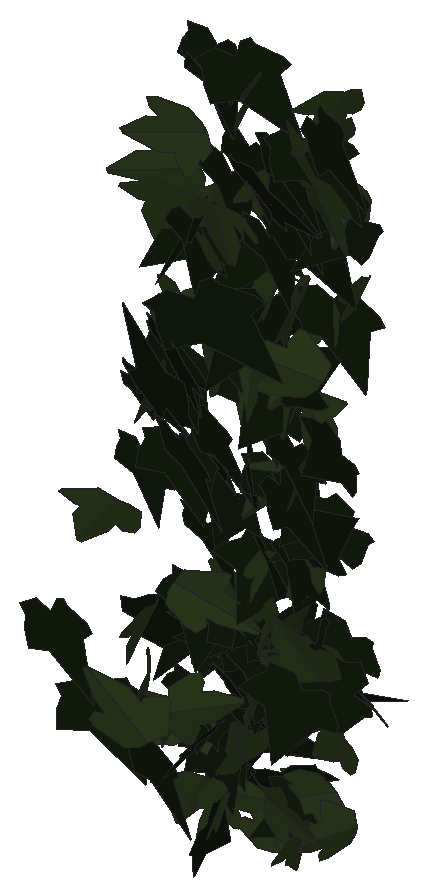
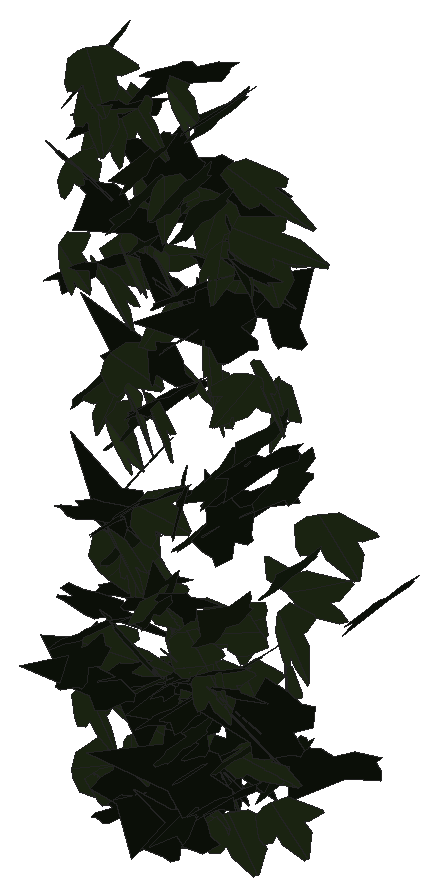
# SketchUp Ruby script. Lengths in inches.
U = 1.inch
M = Sketchup.active_model
def pt(a) = Geom::Point3d.new(a.map { |v| v * U })
def face(e, loops, mat)
  f = e.add_face(loops[0].map { |a| pt(a) })
  loops[1..].each { |l| e.add_face(l.map { |a| pt(a) }).erase! }
  f.material = f.back_material = mat if mat
  f
end
# faces: each face lists its corners as indices into pts; further lists are holes
def faces(e, pts, list, mat = nil) = list.each { |f| face(e, (f[0].is_a?(Array) ? f : [f]).map { |l| l.map { |i| pts[i] } }, mat) }
# xy, xz, yz: faces in a plane at the given z, y or x. An outline is a flat list of corners, or four numbers for a rectangle; further outlines are holes
def ring(l) = l.size == 4 ? [[l[0], l[1]], [l[2], l[1]], [l[2], l[3]], [l[0], l[3]]] : l.each_slice(2).to_a
def flat(e, list, mat, &to3) = list.each { |f| face(e, (f[0].is_a?(Array) ? f : [f]).map { |l| ring(l).map { |u, v| to3.(u, v) } }, mat) }
def xy(e, z, list, mat = nil) = flat(e, list, mat) { |x, y| [x, y, z] }
def xz(e, y, list, mat = nil) = flat(e, list, mat) { |x, z| [x, y, z] }
def yz(e, x, list, mat = nil) = flat(e, list, mat) { |y, z| [x, y, z] }
def lines(e, pts, list) = list.each { |a, b| e.add_line(pt(pts[a]), pt(pts[b])) }
# prism: a flat outline (further loops are holes) pulled along v
def prism(e, loops, v, mat = nil)
  f = face(e, loops, mat); d = Geom::Vector3d.new(v.map { |x| x * U })
  f.pushpull(f.normal.samedirection?(d) ? d.length : -d.length)
end
def box(e, o, s, mat = nil) = prism(e, [[o, [o[0] + s[0], o[1], o[2]], [o[0] + s[0], o[1] + s[1], o[2]], [o[0], o[1] + s[1], o[2]]]], [0, 0, s[2]], mat)
def at(x, y, z, deg = 0) = Geom::Transformation.translation(pt([x, y, z])) * Geom::Transformation.rotation(ORIGIN, Z_AXIS, deg.degrees)
def axes(o, x, y, z) = Geom::Transformation.new([*x, 0, *y, 0, *z, 0, *pt(o).to_a, 1])
def part(name) = M.definitions.add(name)
# library, detail: a bought-in or finely detailed component or shape, given as its bounding box
def library(name, o, s) = part(name).tap { |d| box(d.entities, o, s) }
def detail(e, o, s) = box(e.add_group.entities, o, s)
def put(e, d, t, mat = nil) = e.add_instance(d, t).tap { |i| i.material = mat if mat }
def group(e, t, mat = nil) = e.add_group.tap { |g| g.transformation = t; g.material = mat if mat }.entities
root = M.entities
M.materials.add("1026 AP 7946 SUNNY SIDE UP").color = [254, 231, 186]
M.materials.add("efeu1").color = [18, 25, 13]
M.materials.add("efeu2").color = [43, 57, 29]
c1 = part("ivyleaf_10")
p = [[0,0.5,-0.03],[-0.0625,2.02,-0.43],[-0.19,2.01,-0.46],[-0.54,1.05,-0.29],[-0.52,0.625,-0.18],[-0.83,0.76,-0.28],
  [-1.16,0.64,-0.33],[-1.15,0.33,-0.24],[-0.77,-0.39,0.02],[-0.3,-0.51,0.16],[0.04,-0.48,0.23],[-0.02,2.01,-0.4375],
  [-0.06,2.01,-0.43],[0.04,-0.49,0.23],[0.67,-0.49,0.14],[1.38,0.36,-0.2],[1.375,0.51,-0.24],[0.81,0.65,-0.19],
  [0.62,0.59,-0.15],[0.6,1.09,-0.28],[0.5,1.23,-0.31]]
faces(c1.entities,p,[[0,1,2,3,4,5,6,7,8,9,10],[11,12,0,13,14,15,16,17,18,19,20]],"efeu2")
c2 = part("ivyleaf_9")
p = [[1.54,2.16,1.25],[1.36,2.04,1.19],[-0.21,0.99,0.68],[-0.71,1.11,0.82],[-0.85,0.86,0.67],[-0.8,0.17,0.21],
  [-0.9,-0.01,0.1],[-0.67,-0.16,-0.02],[-0.08,-0.08,-0.05],[-0.03,-0.6,-0.4],[0.65,-0.88,-0.66],[0.83,-0.6,-0.49],
  [1.29,-0.42,-0.43],[1.8125,-0.07,-0.26],[1.21,0.44,0.15]]
faces(c2.entities,p,[[0,1,2,3,4,5,6,7,8,9,10,11,12,13,14]],"efeu1")
put(root,c1,axes([125.9,211.91,280.18],[-0.21426,-0.24961,0.13484],[-0.08049,-0.12264,-0.2934],[0.43686,-0.14502,0.01207]),"1026 AP 7946 SUNNY SIDE UP")
put(root,c2,axes([125.66,211.98,283.87],[0.04707,-0.31543,0.10585],[0.0219,-0.10368,-0.32699],[0.52205,0.03279,0.00417]),"1026 AP 7946 SUNNY SIDE UP")
put(root,c1,axes([126.125,210.66,283.84],[-0.41418,-0.14278,0.1658],[-0.19271,-0.11107,-0.30725],[0.27921,-0.28846,0.03389]),"1026 AP 7946 SUNNY SIDE UP")
put(root,c2,axes([125.74,211.64,285.24],[0.41137,-0.17857,-0.12342],[-0.1051,0.11015,-0.3216],[0.32044,0.26537,0.05296]),"1026 AP 7946 SUNNY SIDE UP")
put(root,c2,axes([125.77,210.97,280.66],[-0.12936,-0.29497,-0.23967],[0.15409,0.2113,-0.31272],[0.56858,-0.12438,0.03022]),"1026 AP 7946 SUNNY SIDE UP")
put(root,c1,axes([126.41,211.85,288.63],[-0.15114,-0.01057,0.36615],[-0.42458,-0.23747,-0.08388],[0.36392,-0.28144,0.0542]),"1026 AP 7946 SUNNY SIDE UP")
put(root,c2,axes([125.875,209.73,282.48],[0.15357,-0.35799,-0.09597],[-0.03239,0.08883,-0.38174],[0.57994,0.09976,0.00409]),"1026 AP 7946 SUNNY SIDE UP")
put(root,c1,axes([126.33,211.76,286.52],[0.1888,-0.21894,-0.27075],[-0.22717,0.21856,-0.25551],[0.48587,0.18726,-0.01426]),"1026 AP 7946 SUNNY SIDE UP")
put(root,c2,axes([126.08,212.02,285.5],[0.04043,-0.33743,-0.16447],[-0.00679,0.15783,-0.34762],[0.58564,0.02512,0.00733]),"1026 AP 7946 SUNNY SIDE UP")
put(root,c1,axes([126.64,211.67,289.35],[0.293,-0.09758,-0.33633],[-0.50379,0.07465,-0.2113],[0.17992,0.36793,-0.04394]),"1026 AP 7946 SUNNY SIDE UP")
put(root,c2,axes([125.82,211.83,281.44],[0.26233,0.01004,0.32465],[0.49231,-0.04681,-0.16952],[0.05774,0.35344,-0.02957]),"1026 AP 7946 SUNNY SIDE UP")
put(root,c1,axes([126.53,211.56,288.33],[-0.53792,-0.12889,0.11284],[-0.1416,-0.07234,-0.37536],[0.22602,-0.35208,0.03339]),"1026 AP 7946 SUNNY SIDE UP")
put(root,c2,axes([126.43,212.14,281.53],[-0.43662,0.03839,-0.16325],[0.22799,-0.08593,-0.2833],[-0.11801,-0.30806,0.05671]),"1026 AP 7946 SUNNY SIDE UP")
put(root,c2,axes([126.15,212.01,285.65],[0.11219,-0.3542,0.13675],[0.0355,-0.1329,-0.37298],[0.59483,0.07474,-0.00354]),"1026 AP 7946 SUNNY SIDE UP")
put(root,c1,axes([126.35,211.99,286.46],[-0.29245,-0.24062,-0.16416],[0.27249,0.05658,-0.29863],[0.3614,-0.23738,0.09232]),"1026 AP 7946 SUNNY SIDE UP")
put(root,c1,axes([126.61,210.85,282.27],[0.08597,-0.37699,0.06829],[0.01345,-0.0679,-0.39283],[0.60231,0.05533,-0.00097]),"1026 AP 7946 SUNNY SIDE UP")
put(root,c1,axes([126.68,210.74,281.45],[0.10564,-0.26469,-0.20128],[-0.03103,0.19428,-0.27916],[0.51497,0.06601,0.02447]),"1026 AP 7946 SUNNY SIDE UP")
put(root,c1,axes([126.67,210.91,285.77],[0.01043,-0.27646,-0.24771],[0.01766,0.23896,-0.28319],[0.57424,-0.00233,0.01321]),"1026 AP 7946 SUNNY SIDE UP")
put(root,c1,axes([126.86,211.43,280.51],[0.30086,0.09889,-0.25801],[-0.33829,-0.12976,-0.22237],[-0.25598,0.28771,-0.00938]),"1026 AP 7946 SUNNY SIDE UP")
put(root,c1,axes([126.8,212.17,282.01],[-0.16875,-0.2955,0.11595],[-0.0092,-0.11874,-0.32279],[0.49807,-0.10231,0.03332]),"1026 AP 7946 SUNNY SIDE UP")
put(root,c2,axes([126.96,211.8,288.01],[-0.52918,-0.07609,0.03235],[-0.03598,-0.04235,-0.35375],[0.12461,-0.33538,0.03523]),"1026 AP 7946 SUNNY SIDE UP")
put(root,c2,axes([126.51,212.28,282.96],[0.09016,-0.29168,0.14703],[0.10212,-0.1334,-0.30499],[0.50146,0.07961,0.03568]),"1026 AP 7946 SUNNY SIDE UP")
put(root,c2,axes([126.65,211.57,284.59],[-0.12958,-0.31232,-0.1472],[0.05934,0.13598,-0.33196],[0.53561,-0.09063,0.00117]),"1026 AP 7946 SUNNY SIDE UP")
put(root,c2,axes([126.66,211.96,282.03],[-0.08444,-0.34733,0.15121],[0.0081,-0.1509,-0.36197],[0.59407,-0.04731,0.02643]),"1026 AP 7946 SUNNY SIDE UP")
put(root,c1,axes([126.96,211.53,279.47],[-0.31475,-0.23428,0.10941],[-0.07714,-0.09903,-0.31694],[0.39793,-0.20451,0.0251]),"1026 AP 7946 SUNNY SIDE UP")
put(root,c1,axes([126.79,211.99,288.28],[-0.10063,-0.3401,-0.03506],[0.15434,0.01297,-0.34313],[0.51449,-0.07041,0.09608]),"1026 AP 7946 SUNNY SIDE UP")
put(root,c1,axes([126.89,212.1,286.9],[0.05887,-0.34036,-0.10486],[0.01883,0.10157,-0.35142],[0.55742,0.03251,0.02295]),"1026 AP 7946 SUNNY SIDE UP")
put(root,c2,axes([126.94,211.55,288.24],[-0.34851,0.15259,-0.2622],[0.29811,-0.17298,-0.27699],[-0.36049,-0.29056,0.02444]),"1026 AP 7946 SUNNY SIDE UP")
put(root,c2,axes([126.56,212.0625,284.15],[0.41505,-0.11879,-0.17574],[0.26803,-0.03222,0.29582],[-0.18555,-0.31226,0.03422]),"1026 AP 7946 SUNNY SIDE UP")
put(root,c2,axes([126.61,210.85,280.17],[0.25311,-0.34619,0.02628],[-0.00276,-0.03109,-0.3932],[0.54605,0.16031,-0.01417]),"1026 AP 7946 SUNNY SIDE UP")
put(root,c2,axes([126.74,211.81,280.67],[-0.05678,-0.28883,0.1652],[0.0277,-0.1644,-0.29888],[0.51998,-0.02278,0.03396]),"1026 AP 7946 SUNNY SIDE UP")
put(root,c1,axes([126.85,211.58,287.78],[-0.41219,0.21266,-0.08037],[0.05824,-0.07932,-0.34608],[-0.35205,-0.26211,0.03684]),"1026 AP 7946 SUNNY SIDE UP")
put(root,c2,axes([126.71,211.98,280.1875],[0.07354,-0.30815,-0.09412],[0.02086,0.09234,-0.31944],[0.50418,0.04112,0.02694]),"1026 AP 7946 SUNNY SIDE UP")
put(root,c2,axes([126.92,212.15,281.8],[-0.36679,-0.21363,-0.04625],[0.10572,-0.00963,-0.32148],[0.32616,-0.23712,0.0522]),"1026 AP 7946 SUNNY SIDE UP")
put(root,c2,axes([126.51,212.05,287.36],[0.42447,-0.00759,0.22204],[0.33911,0.01643,-0.27752],[-0.00681,0.34507,0.02013]),"1026 AP 7946 SUNNY SIDE UP")
put(root,c1,axes([127.18,211.61,285.92],[0.03021,-0.00244,-0.37477],[-0.24899,0.3279,-0.00896],[0.51497,0.15868,0.01766]),"1026 AP 7946 SUNNY SIDE UP")
put(root,c1,axes([127.26,212.04,282.29],[-0.37935,0.0735,0.23987],[-0.37344,0.00281,-0.25487],[-0.08637,-0.33499,0.04843]),"1026 AP 7946 SUNNY SIDE UP")
put(root,c2,axes([126.79,212.12,290.5],[-0.01189,-0.34847,0.07198],[0.00196,-0.07189,-0.35949],[0.55946,-0.00715,0.00279]),"1026 AP 7946 SUNNY SIDE UP")
put(root,c2,axes([126.9,211.66,287.88],[-0.02053,-0.31755,0.21286],[-0.0241,-0.20794,-0.32858],[0.59677,-0.01932,-0.00594]),"1026 AP 7946 SUNNY SIDE UP")
put(root,c2,axes([127.125,212.21,281.9],[-0.31569,-0.24526,0.14014],[-0.07183,-0.13817,-0.32359],[0.43619,-0.20026,0.04814]),"1026 AP 7946 SUNNY SIDE UP")
put(root,c2,axes([126.85,211.99,290.33],[0.07159,-0.33275,0.10543],[0.03972,-0.10169,-0.34641],[0.54684,0.05095,0.01136]),"1026 AP 7946 SUNNY SIDE UP")
put(root,c1,axes([126.9,211.92,281.87],[0.20417,0.23732,0.19125],[0.16186,0.15348,-0.27743],[-0.44387,0.16513,-0.0132]),"1026 AP 7946 SUNNY SIDE UP")
put(root,c2,axes([126.84,211.78,284.9],[0.31395,-0.31377,-0.03146],[-0.03224,0.02103,-0.38297],[0.49439,0.20062,-0.005]),"1026 AP 7946 SUNNY SIDE UP")
put(root,c1,axes([127.24,210.82,281.21],[0.03761,-0.38204,0.05583],[0.00268,-0.05637,-0.39467],[0.60722,0.02391,-0.00171]),"1026 AP 7946 SUNNY SIDE UP")
put(root,c2,axes([127.3125,211.2,280.48],[-0.22647,0.19756,-0.21128],[0.14467,-0.18653,-0.2514],[-0.42509,-0.16873,0.027]),"1026 AP 7946 SUNNY SIDE UP")
put(root,c2,axes([127.59,211.84,281.79],[-0.39332,0.21224,0.11918],[-0.17616,0.04379,-0.33555],[-0.33578,-0.27158,0.03644]),"1026 AP 7946 SUNNY SIDE UP")
put(root,c2,axes([127.23,212.27,287.01],[-0.21043,-0.20198,0.28859],[-0.10601,-0.28058,-0.24226],[0.53408,-0.13528,0.06562]),"1026 AP 7946 SUNNY SIDE UP")
put(root,c1,axes([126.87,211.47,282.4],[0.17157,0.11682,0.33616],[0.43237,0.17793,-0.15963],[-0.33013,0.29375,-0.03437]),"1026 AP 7946 SUNNY SIDE UP")
put(root,c2,axes([127.29,212.24,287.64],[-0.21923,-0.28492,0.14128],[-0.04982,-0.1383,-0.32616],[0.49581,-0.13988,0.0297]),"1026 AP 7946 SUNNY SIDE UP")
put(root,c2,axes([127.15,211.79,280.46],[0.02541,-0.31283,-0.04939],[0.00441,0.04637,-0.32239],[0.4972,0.01558,0.00538]),"1026 AP 7946 SUNNY SIDE UP")
put(root,c2,axes([127.11,212.03,288.7],[0.02188,-0.31138,0.19306],[0.04089,-0.18797,-0.32182],[0.57142,0.02537,0.01564]),"1026 AP 7946 SUNNY SIDE UP")
put(root,c2,axes([127.25,211.9,283.88],[-0.13291,-0.26682,0.21314],[-0.00672,-0.21395,-0.28521],[0.53231,-0.06932,0.04962]),"1026 AP 7946 SUNNY SIDE UP")
put(root,c2,axes([127.58,210.01,286.23],[0.22051,-0.18211,0.37102],[-0.22428,0.33545,0.23326],[-0.59517,-0.19388,0.04956]),"1026 AP 7946 SUNNY SIDE UP")
put(root,c2,axes([127.23,212.11,281.84],[0.00985,-0.31605,-0.07882],[0.00526,0.07479,-0.32519],[0.51064,0.00533,0.00487]),"1026 AP 7946 SUNNY SIDE UP")
put(root,c2,axes([127.24,212.26,280.88],[-0.00424,-0.27285,0.17992],[0.04292,-0.17577,-0.28101],[0.5089,0.01255,0.0252]),"1026 AP 7946 SUNNY SIDE UP")
put(root,c1,axes([127.45,211.34,288.5],[-0.53448,0.08056,-0.02626],[0.02721,-0.03898,-0.35841],[-0.13027,-0.33866,0.03289]),"1026 AP 7946 SUNNY SIDE UP")
put(root,c1,axes([127.76,209.18,281.66],[0.42812,0.09371,0.27639],[-0.42494,-0.02715,0.29273],[0.13561,-0.3809,0.04475]),"1026 AP 7946 SUNNY SIDE UP")
put(root,c2,axes([127.29,212.1875,289.08],[0.08936,-0.32492,0.12848],[0.04398,-0.12357,-0.34048],[0.54652,0.06307,0.00639]),"1026 AP 7946 SUNNY SIDE UP")
put(root,c2,axes([127.32,211.49,280.23],[-0.21941,-0.12673,-0.2633],[0.44049,-0.01094,-0.15247],[0.07917,-0.29036,0.11864]),"1026 AP 7946 SUNNY SIDE UP")
put(root,c2,axes([127.19,211.87,280.92],[0.23662,-0.19636,0.20419],[0.16661,-0.16946,-0.2554],[0.40718,0.18345,-0.01415]),"1026 AP 7946 SUNNY SIDE UP")
put(root,c2,axes([127.4,212.27,281.4],[-0.04643,-0.32901,0.02111],[0.00186,-0.02255,-0.34042],[0.51853,-0.02938,0.00311]),"1026 AP 7946 SUNNY SIDE UP")
put(root,c2,axes([127.67,211.85,284.06],[-0.0374,-0.14211,0.31392],[0.06292,0.30293,0.15014],[-0.52608,0.04633,-0.00436]),"1026 AP 7946 SUNNY SIDE UP")
put(root,c2,axes([127.24,212.13,281.57],[0.41293,-0.1938,0.04894],[0.03696,-0.04975,-0.33547],[0.31198,0.2624,-0.02503]),"1026 AP 7946 SUNNY SIDE UP")
put(root,c2,axes([127.125,211.9375,280.38],[0.24028,0.01978,-0.37834],[0.40972,0.275,0.12853],[0.40838,-0.28755,0.09366]),"1026 AP 7946 SUNNY SIDE UP")
put(root,c2,axes([127.45,211.91,279.79],[0.44163,-0.17695,-0.0857],[-0.13433,0.01796,-0.34053],[0.2758,0.29209,-0.02863]),"1026 AP 7946 SUNNY SIDE UP")
put(root,c1,axes([127.27,211.6,279.5],[0.0933,-0.10817,-0.33715],[0.46805,-0.15016,0.10605],[-0.27144,-0.2961,0.06698]),"1026 AP 7946 SUNNY SIDE UP")
put(root,c1,axes([127.64,211.87,290.33],[0.18623,-0.28707,0.19375],[0.08651,-0.18225,-0.32057],[0.53409,0.12961,-0.01564]),"1026 AP 7946 SUNNY SIDE UP")
put(root,c2,axes([127.72,212.2,282.89],[-0.37242,-0.23772,0.00826],[0.01501,-0.0227,-0.34504],[0.37377,-0.23595,0.02209]),"1026 AP 7946 SUNNY SIDE UP")
put(root,c2,axes([127.62,209.98,287.21],[0.52573,-0.13376,-0.23911],[-0.36534,0.03755,-0.36808],[0.20759,0.40484,-0.04222]),"1026 AP 7946 SUNNY SIDE UP")
put(root,c1,axes([127.74,212.11,282.86],[0.17817,0.26073,-0.16487],[-0.12168,-0.14231,-0.29342],[-0.46665,0.13666,0.01356]),"1026 AP 7946 SUNNY SIDE UP")
put(root,c1,axes([127.83,212.23,284.19],[-0.09572,-0.19528,0.28607],[-0.0144,-0.28218,-0.20733],[0.53503,-0.04253,0.0456]),"1026 AP 7946 SUNNY SIDE UP")
put(root,c2,axes([127.48,211.71,290.73],[0.0812,-0.30108,-0.23651],[0.10677,0.23364,-0.30082],[0.58404,-0.00085,0.08788]),"1026 AP 7946 SUNNY SIDE UP")
put(root,c1,axes([127.75,211.96,288.89],[-0.06792,-0.34814,-0.01351],[0.1146,0.00194,-0.35369],[0.53557,-0.04456,0.07396]),"1026 AP 7946 SUNNY SIDE UP")
put(root,c2,axes([127.91,210.53,279.59],[-0.00399,-0.04884,-0.40501],[-0.41575,0.29262,-0.034],[0.46331,0.26216,-0.034]),"1026 AP 7946 SUNNY SIDE UP")
put(root,c2,axes([127.52,212,279.24],[-0.09505,-0.00684,0.34056],[0.48079,-0.12917,0.05409],[0.19804,0.31029,0.03215]),"1026 AP 7946 SUNNY SIDE UP")
put(root,c1,axes([127.86,210.78,279.88],[0.37158,-0.31751,0.0587],[0.02555,-0.06106,-0.40741],[0.50709,0.23574,-0.02248]),"1026 AP 7946 SUNNY SIDE UP")
put(root,c2,axes([127.98,211.41,286.97],[-0.53008,-0.00235,-0.14834],[0.22465,-0.05138,-0.34404],[-0.02837,-0.36295,0.0475]),"1026 AP 7946 SUNNY SIDE UP")
put(root,c2,axes([127.72,212.26,282.76],[-0.02893,-0.16298,0.296],[0.04528,-0.28839,-0.16777],[0.5187,0.01608,0.03116]),"1026 AP 7946 SUNNY SIDE UP")
put(root,c2,axes([127.73,211.92,285.81],[-0.03524,-0.37579,-0.01596],[0.02188,0.01254,-0.38752],[0.59086,-0.02288,0.0134]),"1026 AP 7946 SUNNY SIDE UP")
put(root,c1,axes([127.75,211.6,286.12],[0.43931,-0.16634,0.17307],[0.19439,-0.12059,-0.33364],[0.3181,0.30341,-0.03514]),"1026 AP 7946 SUNNY SIDE UP")
put(root,c1,axes([127.97,211.93,286.63],[-0.0528,0.31089,0.19834],[0.0428,-0.1889,0.32098],[0.57194,0.04284,-0.00571]),"1026 AP 7946 SUNNY SIDE UP")
put(root,c1,axes([128.01,211.92,285.58],[0.34497,-0.24273,-0.09955],[-0.08211,0.08106,-0.33624],[0.4017,0.22502,0.01676]),"1026 AP 7946 SUNNY SIDE UP")
put(root,c2,axes([127.79,212.15,284.35],[0.00684,-0.32615,-0.08804],[0.01986,0.08372,-0.33525],[0.52904,0.00107,0.01373]),"1026 AP 7946 SUNNY SIDE UP")
put(root,c2,axes([128.01,211.9,285.64],[-0.22516,-0.26214,0.19597],[-0.07318,-0.19079,-0.30569],[0.50539,-0.14441,0.04304]),"1026 AP 7946 SUNNY SIDE UP")
put(root,c1,axes([127.82,210.08,281.57],[0.01907,-0.0578,-0.39767],[0.34064,0.32187,-0.04079],[0.50992,-0.21285,0.04212]),"1026 AP 7946 SUNNY SIDE UP")
put(root,c2,axes([127.96,211.86,281.43],[-0.16673,-0.26976,0.16066],[0.02254,-0.17034,-0.29164],[0.49064,-0.08385,0.06799]),"1026 AP 7946 SUNNY SIDE UP")
put(root,c2,axes([128.08,211.93,279.85],[0.28533,0.25877,-0.05011],[-0.02739,-0.04893,-0.32558],[-0.41354,0.18178,-0.01301]),"1026 AP 7946 SUNNY SIDE UP")
put(root,c1,axes([128.19,211.64,279.03],[0.44212,0.07542,0.12862],[-0.20053,-0.00254,0.29848],[0.11011,-0.30746,0.02717]),"1026 AP 7946 SUNNY SIDE UP")
put(root,c1,axes([128.11,211.57,287.46],[0.28857,-0.29342,0.02424],[-0.00875,-0.03314,-0.356],[0.463,0.18226,-0.02183]),"1026 AP 7946 SUNNY SIDE UP")
put(root,c1,axes([128.16,212.13,285.67],[0.25888,-0.29879,-0.0069],[-0.0186,-0.00081,-0.35128],[0.46952,0.16472,-0.01011]),"1026 AP 7946 SUNNY SIDE UP")
put(root,c2,axes([127.93,212.06,289.33],[0.2394,-0.3377,0.01791],[-0.00755,-0.02332,-0.38148],[0.53181,0.15169,-0.01348]),"1026 AP 7946 SUNNY SIDE UP")
put(root,c2,axes([127.8125,211.64,288.89],[0.21132,-0.16958,0.30668],[0.28359,-0.23808,-0.22427],[0.45957,0.22489,-0.00263]),"1026 AP 7946 SUNNY SIDE UP")
put(root,c2,axes([128.37,212.18,282.18],[-0.44833,0.06841,-0.1663],[0.21999,-0.09813,-0.29729],[-0.16706,-0.31281,0.0548]),"1026 AP 7946 SUNNY SIDE UP")
put(root,c1,axes([128.62,211.59,289.72],[-0.22815,0.07903,0.32269],[-0.47309,0.09063,-0.16684],[-0.18308,-0.33267,0.02901]),"1026 AP 7946 SUNNY SIDE UP")
put(root,c2,axes([128.03,212.18,288.71],[0.16745,-0.34565,0.0491],[0.00033,-0.05182,-0.37259],[0.54908,0.10545,-0.01475]),"1026 AP 7946 SUNNY SIDE UP")
put(root,c2,axes([128.03,211.72,288.14],[0.09765,-0.33352,0.12872],[0.04335,-0.12388,-0.35019],[0.5594,0.06782,0.00467]),"1026 AP 7946 SUNNY SIDE UP")
put(root,c1,axes([128.39,212.07,286.16],[-0.17001,-0.20832,0.26366],[-0.02877,-0.26631,-0.23177],[0.51954,-0.08292,0.07345]),"1026 AP 7946 SUNNY SIDE UP")
put(root,c1,axes([128.375,211.29,282.6],[0.2059,-0.31581,-0.08167],[-0.03075,0.07573,-0.35159],[0.51038,0.13197,0.01176]),"1026 AP 7946 SUNNY SIDE UP")
put(root,c2,axes([128.31,212.375,283.95],[-0.18684,-0.2456,0.22459],[-0.09019,-0.21425,-0.28033],[0.50992,-0.12788,0.03271]),"1026 AP 7946 SUNNY SIDE UP")
put(root,c2,axes([128.16,211.46,287.27],[-0.32896,-0.0831,-0.28705],[0.44588,0.01497,-0.22424],[0.09782,-0.34774,0.05679]),"1026 AP 7946 SUNNY SIDE UP")
put(root,c2,axes([128.56,211.93,281.34],[-0.31662,-0.12994,0.21871],[-0.26116,-0.13452,-0.24704],[0.29285,-0.26046,0.01616]),"1026 AP 7946 SUNNY SIDE UP")
put(root,c1,axes([128.375,210.76,280.76],[-0.13245,-0.29257,-0.18275],[-0.09806,-0.16477,0.31242],[-0.52762,0.10407,-0.01219]),"1026 AP 7946 SUNNY SIDE UP")
put(root,c2,axes([128.53,212.05,279.43],[-0.28769,-0.17217,0.19967],[-0.20157,-0.14748,-0.25919],[0.35563,-0.22287,0.01461]),"1026 AP 7946 SUNNY SIDE UP")
put(root,c1,axes([128.79,211.98,281.71],[0.10144,-0.01686,-0.36928],[-0.56402,-0.00944,-0.06612],[-0.00993,0.364,-0.01668]),"1026 AP 7946 SUNNY SIDE UP")
put(root,c1,axes([128.3,211.09,281.52],[0.18646,-0.22358,0.27431],[0.18234,-0.24121,-0.26203],[0.51703,0.1657,-0.00652]),"1026 AP 7946 SUNNY SIDE UP")
put(root,c1,axes([128.68,211.98,279.73],[0.30615,-0.03301,-0.26486],[-0.4031,0.02145,-0.20286],[0.0583,0.32164,-0.01175]),"1026 AP 7946 SUNNY SIDE UP")
put(root,c2,axes([128.09,209.69,285.93],[0.24693,-0.34626,0.14039],[0.05556,-0.13551,-0.3918],[0.58361,0.15941,-0.0221]),"1026 AP 7946 SUNNY SIDE UP")
put(root,c2,axes([128.13,211.77,285.99],[-0.17633,0.10078,0.34807],[0.44299,-0.18656,0.15283],[0.3319,0.30255,-0.01906]),"1026 AP 7946 SUNNY SIDE UP")
put(root,c2,axes([128.2,209.95,288.03],[-0.09139,-0.15077,-0.41258],[0.26984,0.36109,-0.16394],[0.61502,-0.18083,0.01062]),"1026 AP 7946 SUNNY SIDE UP")
put(root,c2,axes([128.33,211.6,284.47],[0.25738,-0.30073,-0.14654],[-0.12438,0.11685,-0.3518],[0.50691,0.18136,-0.01192]),"1026 AP 7946 SUNNY SIDE UP")
put(root,c1,axes([128.59,211.93,283.36],[0.40372,-0.23231,-0.04311],[-0.07313,0.00885,-0.35576],[0.36351,0.25978,-0.0237]),"1026 AP 7946 SUNNY SIDE UP")
put(root,c2,axes([128.66,211.35,281.01],[0.13482,0.30959,-0.04269],[-0.00816,-0.04337,-0.33113],[-0.49144,0.08565,-0.00621]),"1026 AP 7946 SUNNY SIDE UP")
put(root,c1,axes([128.5625,211.73,287.56],[0.22913,-0.29361,0.11755],[0.07703,-0.10493,-0.33828],[0.49026,0.15371,-0.00179]),"1026 AP 7946 SUNNY SIDE UP")
put(root,c2,axes([128.44,211.73,285.05],[0.07489,-0.32098,0.10646],[0.0267,-0.10379,-0.3349],[0.53044,0.05054,0.00182]),"1026 AP 7946 SUNNY SIDE UP")
put(root,c2,axes([128.53,211.86,283.22],[-0.07632,-0.24015,0.24511],[0.00193,-0.24185,-0.2512],[0.53306,-0.0335,0.036]),"1026 AP 7946 SUNNY SIDE UP")
put(root,c1,axes([128.63,211.89,284.99],[0.22447,-0.31476,0.1926],[0.08057,-0.18344,-0.35615],[0.57144,0.14951,-0.02544]),"1026 AP 7946 SUNNY SIDE UP")
put(root,c1,axes([128.76,211.92,287.25],[0.43579,-0.19977,-0.0625],[-0.08355,0.02808,-0.35169],[0.31695,0.28208,-0.00676]),"1026 AP 7946 SUNNY SIDE UP")
put(root,c1,axes([128.67,211.88,285.62],[0.02322,0.33214,0.1063],[-0.03551,0.1021,-0.34087],[-0.54485,0.0075,0.02675]),"1026 AP 7946 SUNNY SIDE UP")
put(root,c2,axes([128.95,212.18,283.84],[-0.45279,-0.11184,0.11115],[-0.13637,-0.07444,-0.31653],[0.20359,-0.29859,0.03518]),"1026 AP 7946 SUNNY SIDE UP")
put(root,c2,axes([128.43,211.92,288.43],[-0.18614,-0.1222,-0.33908],[0.45052,0.16587,-0.16899],[0.31729,-0.30721,0.04103]),"1026 AP 7946 SUNNY SIDE UP")
put(root,c1,axes([128.8125,211.29,282.81],[-0.03184,-0.33717,-0.10338],[0.01371,0.09808,-0.34739],[0.55213,-0.02188,0.00266]),"1026 AP 7946 SUNNY SIDE UP")
put(root,c1,axes([128.85,212.02,289.94],[-0.14538,-0.36132,-0.03006],[0.02735,0.02354,-0.38392],[0.56908,-0.09343,0.01077]),"1026 AP 7946 SUNNY SIDE UP")
put(root,c2,axes([128.51,211.89,283.62],[-0.12414,0.07629,0.38558],[0.31908,-0.31489,0.10851],[0.50806,0.21641,0.02606]),"1026 AP 7946 SUNNY SIDE UP")
put(root,c1,axes([128.92,212.06,290.46],[-0.22562,-0.3239,0.04203],[-0.00755,-0.04447,-0.36495],[0.51363,-0.14293,0.0131]),"1026 AP 7946 SUNNY SIDE UP")
put(root,c1,axes([129.13,211.86,280.74],[-0.31229,0.12106,0.2335],[-0.36278,0.0402,-0.23086],[-0.17573,-0.29815,0.06162]),"1026 AP 7946 SUNNY SIDE UP")
put(root,c2,axes([128.6,211.78,289.81],[0.0435,-0.31312,-0.20175],[0.11018,0.19553,-0.31358],[0.56867,-0.01393,0.07619]),"1026 AP 7946 SUNNY SIDE UP")
put(root,c1,axes([129.21,210.91,286.86],[0.13584,0.14906,0.37217],[-0.38295,-0.26772,0.17264],[0.47901,-0.2563,0.03248]),"1026 AP 7946 SUNNY SIDE UP")
put(root,c2,axes([128.9,212.33,282.03],[-0.18046,-0.29083,0.10582],[-0.02213,-0.1063,-0.32172],[0.48535,-0.11298,0.02468]),"1026 AP 7946 SUNNY SIDE UP")
put(root,c2,axes([128.625,211.9,281.27],[0.33198,-0.01174,0.24859],[0.36143,0.10868,-0.20105],[-0.11727,0.3017,0.08409]),"1026 AP 7946 SUNNY SIDE UP")
put(root,c1,axes([129.31,211.01,282.29],[-0.4878,-0.01732,-0.18904],[-0.28928,0.01071,0.31961],[-0.01486,0.36022,-0.01648]),"1026 AP 7946 SUNNY SIDE UP")
put(root,c1,axes([129.09,210.96,279.63],[-0.0145,-0.30812,-0.10556],[0.02228,0.10028,-0.31679],[0.50922,-0.01316,0.01085]),"1026 AP 7946 SUNNY SIDE UP")
put(root,c1,axes([129.12,210.82,287.85],[0.12989,-0.33021,-0.09683],[-0.00666,0.09376,-0.34963],[0.53901,0.08073,0.01902]),"1026 AP 7946 SUNNY SIDE UP")
put(root,c1,axes([129.0625,212.22,288.92],[-0.16395,-0.21573,0.26291],[0.14473,-0.27667,-0.20285],[0.50666,0.00922,0.14302]),"1026 AP 7946 SUNNY SIDE UP")
put(root,c1,axes([128.76,210.89,280.01],[0.02226,-0.03553,0.33199],[0.49958,-0.06372,-0.02197],[0.10311,0.31642,0.0348]),"1026 AP 7946 SUNNY SIDE UP")
put(root,c2,axes([129.38,211.97,288.79],[-0.5556,0.10195,-0.07331],[0.093,-0.05271,-0.37758],[-0.17255,-0.35668,0.03254]),"1026 AP 7946 SUNNY SIDE UP")
put(root,c1,axes([129.02,211.56,289.29],[-0.41144,0.20183,-0.17254],[0.17606,-0.12976,-0.33973],[-0.3742,-0.28296,0.02988]),"1026 AP 7946 SUNNY SIDE UP")
put(root,c2,axes([128.83,212.29,281.55],[0.1698,-0.22581,0.22125],[0.17197,-0.18682,-0.25856],[0.46033,0.15309,0.01498]),"1026 AP 7946 SUNNY SIDE UP")
put(root,c2,axes([128.95,211.95,287.39],[-0.02772,-0.36912,-0.1059],[0.07205,0.09804,-0.37793],[0.59729,-0.02896,0.04067]),"1026 AP 7946 SUNNY SIDE UP")
put(root,c1,axes([129.16,212.25,287.57],[0.09686,-0.30005,0.16577],[0.06878,-0.15694,-0.31631],[0.53221,0.07489,0.01071]),"1026 AP 7946 SUNNY SIDE UP")
put(root,c2,axes([129.21,211.72,285.25],[-0.20599,-0.14613,0.29678],[-0.0669,-0.30119,-0.17857],[0.50467,-0.09957,0.09746]),"1026 AP 7946 SUNNY SIDE UP")
put(root,c1,axes([129.32,211.62,279.55],[-0.00029,-0.03193,0.3757],[-0.03162,-0.36432,-0.03499],[0.57504,-0.02005,-0.00173]),"1026 AP 7946 SUNNY SIDE UP")
put(root,c2,axes([129.67,211.38,281.87],[-0.48183,0.0339,0.18172],[-0.28089,-0.02486,-0.31526],[-0.02652,-0.3526,0.03761]),"1026 AP 7946 SUNNY SIDE UP")
put(root,c2,axes([129.27,210.82,281.99],[-0.29843,-0.29899,0.03165],[0.00298,-0.03953,-0.36432],[0.47288,-0.18844,0.02228]),"1026 AP 7946 SUNNY SIDE UP")
put(root,c2,axes([129.1,211.46,290.34],[0.3127,-0.29579,-0.17501],[-0.18013,0.12525,-0.36571],[0.50381,0.22837,-0.02213]),"1026 AP 7946 SUNNY SIDE UP")
